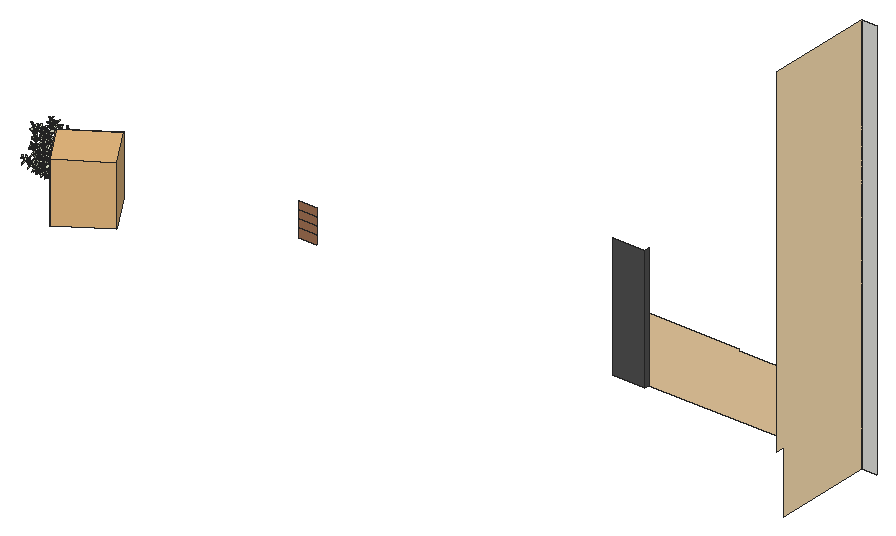
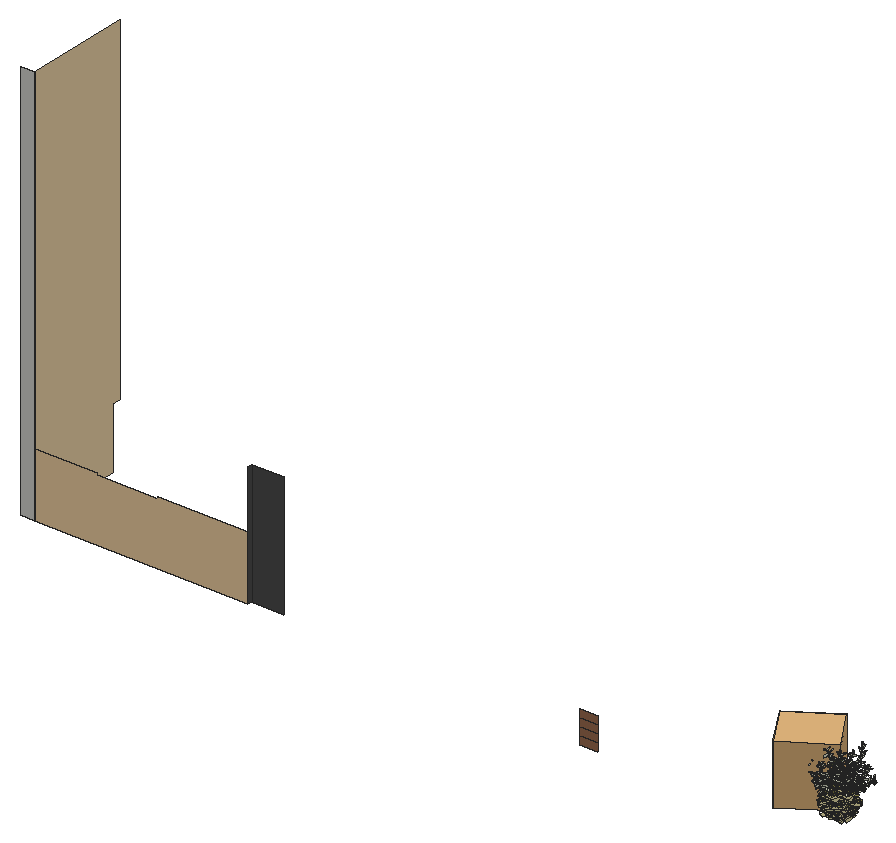
# SketchUp Ruby script. Lengths in inches.
U = 1.inch
M = Sketchup.active_model
def pt(a) = Geom::Point3d.new(a.map { |v| v * U })
def face(e, loops, mat)
  f = e.add_face(loops[0].map { |a| pt(a) })
  loops[1..].each { |l| e.add_face(l.map { |a| pt(a) }).erase! }
  f.material = f.back_material = mat if mat
  f
end
# faces: each face lists its corners as indices into pts; further lists are holes
def faces(e, pts, list, mat = nil) = list.each { |f| face(e, (f[0].is_a?(Array) ? f : [f]).map { |l| l.map { |i| pts[i] } }, mat) }
# xy, xz, yz: faces in a plane at the given z, y or x. An outline is a flat list of corners, or four numbers for a rectangle; further outlines are holes
def ring(l) = l.size == 4 ? [[l[0], l[1]], [l[2], l[1]], [l[2], l[3]], [l[0], l[3]]] : l.each_slice(2).to_a
def flat(e, list, mat, &to3) = list.each { |f| face(e, (f[0].is_a?(Array) ? f : [f]).map { |l| ring(l).map { |u, v| to3.(u, v) } }, mat) }
def xy(e, z, list, mat = nil) = flat(e, list, mat) { |x, y| [x, y, z] }
def xz(e, y, list, mat = nil) = flat(e, list, mat) { |x, z| [x, y, z] }
def yz(e, x, list, mat = nil) = flat(e, list, mat) { |y, z| [x, y, z] }
def lines(e, pts, list) = list.each { |a, b| e.add_line(pt(pts[a]), pt(pts[b])) }
# prism: a flat outline (further loops are holes) pulled along v
def prism(e, loops, v, mat = nil)
  f = face(e, loops, mat); d = Geom::Vector3d.new(v.map { |x| x * U })
  f.pushpull(f.normal.samedirection?(d) ? d.length : -d.length)
end
def box(e, o, s, mat = nil) = prism(e, [[o, [o[0] + s[0], o[1], o[2]], [o[0] + s[0], o[1] + s[1], o[2]], [o[0], o[1] + s[1], o[2]]]], [0, 0, s[2]], mat)
def at(x, y, z, deg = 0) = Geom::Transformation.translation(pt([x, y, z])) * Geom::Transformation.rotation(ORIGIN, Z_AXIS, deg.degrees)
def axes(o, x, y, z) = Geom::Transformation.new([*x, 0, *y, 0, *z, 0, *pt(o).to_a, 1])
def part(name) = M.definitions.add(name)
# library, detail: a bought-in or finely detailed component or shape, given as its bounding box
def library(name, o, s) = part(name).tap { |d| box(d.entities, o, s) }
def detail(e, o, s) = box(e.add_group.entities, o, s)
def put(e, d, t, mat = nil) = e.add_instance(d, t).tap { |i| i.material = mat if mat }
def group(e, t, mat = nil) = e.add_group.tap { |g| g.transformation = t; g.material = mat if mat }.entities
root = M.entities
M.materials.add("0ad16as01f6asdLeafVar1sfd015as60f1as6").color = [231, 235, 211]
M.materials.add("Colorsadfasdfa0sd1f06w3").color = [153, 130, 61]
M.materials.add("Euphorbia asdfasd0f150160s159w").color = [180, 173, 131]
M.materials.add("Euphorbiaasdfa0sdf1a56sd016wow Leaf SU").color = [141, 134, 72]
M.materials.add("[0032_Moccasin]").color = [255, 228, 181]
M.materials.add("[0033_NavajoWhite]").color = [255, 222, 173]
M.materials.add("[0135_DarkGray]").color = [81, 81, 81]
M.materials.add("[Tile Ceramic Multi]").color = [165, 115, 84]
M.materials.add("asdfasdf0165f6asdLeafVar1sfd015as60f1as6").color = [231, 235, 211]
M.materials.add("dw_stemssadfasdfa0sdf1s01d6w1").color = [90, 97, 50]
M.materials.add("viburnumbladsadfasdfad0w122").color = [125, 129, 119]
c1 = part("Component\#315")
p = [[0.25,0,0],[2.05,0.01,0.35],[1.81,4.2,1.66],[0,4.19,1.3125]]
faces(c1.entities,p,[[0,1,2,3]],"viburnumbladsadfasdfad0w122")
c2 = part("viburnumblad2")
put(c2.entities,c1,axes([-19.23,-4.49,-32.18],[83.35428,0,0],[0,79.38502,0],[0,0,83.35428]))
c3 = part("vdw_leaf\#2")
p = [[0,0,0],[-2.77,1.61,2.32],[-4.3125,6.1,4.5],[-3.97,13.49,6.09],[-2.47,18.57,6.3],[-0.2,22.73,5.75],
  [2.54,19.66,6.85],[4.3,15.93,7.09],[5.03,7.6,5.43],[3.32,1.76,2.74]]
faces(c3.entities,p,[[0,1,2,3,4,5],[0,5,6,7,8,9]],"asdfasdf0165f6asdLeafVar1sfd015as60f1as6")
c4 = part("dg_branch_1\#2")
p = [[46.12,1.57,35.62],[46,5.42,35.41],[0.14,1.79,0.05],[0.26,-2.0625,0.27],[74.05,2.99,75.8],[74.11,5.28,75.58],
  [103.46,0.47,94.74],[104.03,2.92,94.84],[81.14,16.92,120.46],[81.2,18.78,120.24],[130.47,-5.6875,130.27],[130.58,-3.66,129.85],
  [80.82,34.4375,191.22],[80.64,35.93,190.9],[148.49,-14.56,203.24],[148.9,-12.8125,203.11],[81.08,37.95,226.93],[81.4,39.1,227.03],
  [157.45,-18.19,250.77],[157.7,-17.01,250.41]]
faces(c4.entities,p,[[0,1,2,3],[4,0,1],[4,1,5],[6,4,5],[6,5,7],[8,4,5],[8,5,9],[10,6,7],
  [10,7,11],[12,8,9],[12,9,13],[14,10,11],[14,11,15],[16,12,13],[16,13,17],[18,14,15],
  [18,15,19]],"dw_stemssadfasdfa0sdf1s01d6w1")
c5 = part("vdw_branch1\#3")
put(c5.entities,c3,axes([120.69,-2.42,117.31],[1.12221,-0.24063,-0.65809],[0.19207,1.24776,-0.12871],[0.65778,0.01392,1.11658]))
put(c5.entities,c3,axes([81,38.9,226.05],[0.7888,-0.58155,0],[0.48308,0.65523,0.47],[-0.28484,-0.38635,0.83138]))
put(c5.entities,c3,axes([78.08,12.69,106.05],[-1.43826,-0.02353,-0.03177],[0.0088,-1.31777,0.57755],[-0.03854,0.57714,1.31741]))
put(c5.entities,c3,axes([130.18,-4.73,130.41],[-0.38031,-1.29044,-0.11242],[1.20662,-0.31032,-0.51987],[0.47109,-0.24694,1.24081]))
put(c5.entities,c3,axes([157.08,-17.89,249.93],[-0.91355,0.40674,0],[-0.37496,-0.84216,0.38752],[0.15762,0.35401,0.92186]))
put(c5.entities,c3,axes([90.64,3.03,86.49],[0.32514,-0.85045,-0.99675],[0.69523,0.98247,-0.61148],[1.11061,-0.36604,0.67459]))
put(c5.entities,c3,axes([80.15,28.42,160.95],[-0.16039,0.95636,-1.06292],[-1.41646,0.03966,0.24943],[0.19509,1.07422,0.93709]))
put(c5.entities,c3,axes([126.74,-5.45,129.22],[-0.59819,0.96152,-0.6841],[-0.85772,0.12575,0.92675],[0.75427,0.88089,0.57856]))
put(c5.entities,c3,axes([133.22,-6.12,150.66],[-0.93823,0.76985,0.59124],[-0.47726,-1.08188,0.65135],[0.84525,0.24366,1.02405]))
put(c5.entities,c3,axes([80.43,22.89,141.32],[-1.42571,-0.19312,0.01373],[0.18338,-1.31425,0.5561],[-0.0621,0.5528,1.32692]))
put(c5.entities,c3,axes([33.14,0.88,26.42],[-0.13338,1.31536,0.04876],[-1.04528,-0.13221,0.7073],[0.72315,0.03348,1.07497]))
put(c5.entities,c3,axes([152.63,-15.08,221.76],[-1.28188,0.41945,0.0579],[-0.3638,-1.18547,0.53367],[0.21665,0.49113,1.23869]))
put(c5.entities,c3,axes([80.05,28.28,160.33],[-0.46732,-1.26661,0.40679],[1.27397,-0.40257,0.21004],[-0.07408,0.44645,1.30501]))
put(c5.entities,c3,axes([153.95,-14.8,235.875],[0.39005,1.07743,0.20605],[-0.96443,0.25296,0.50293],[0.42961,-0.3464,0.99807]))
put(c5.entities,c3,axes([80.2,24.22,141.74],[1.33062,-0.46576,0.02628],[0.44746,1.2746,-0.06608],[-0.00197,0.0722,1.37936]))
put(c5.entities,c3,axes([145.48,-12.5,188.92],[-1.32952,0.16983,0.16138],[-0.09299,-1.2361,0.53471],[0.21503,0.51548,1.22904]))
put(c5.entities,c3,axes([139.64,-9.18,171.24],[0.05682,1.30088,0.23414],[-1.13176,-0.05343,0.57151],[0.58357,-0.22963,1.13417]))
put(c5.entities,c3,axes([70.95,4.35,71.98],[-1.1081,-0.41873,0.64752],[0.33675,-1.28259,-0.25313],[0.6937,-0.04625,1.15721]))
put(c5.entities,c3,axes([59.85,4.55,56.17],[-0.26797,1.24526,0.35754],[-0.9369,-0.41634,0.74783],[0.83377,-0.10389,0.98674]))
put(c5.entities,c3,axes([33.11,3.36,25.66],[-0.57817,-1.07968,-0.5679],[1.11554,-0.21356,-0.7297],[0.49375,-0.78178,0.98363]))
put(c5.entities,c4,at(-0.21,0.34,-0.17),"dw_stemssadfasdfa0sdf1s01d6w1")
put(c5.entities,c3,axes([80.91,19.01,122.53],[-0.84258,1.13222,-0.27981],[-1.15093,-0.75138,0.42537],[0.18861,0.47293,1.3457]))
put(c5.entities,c3,axes([119.8,-1.22,114.1],[-1.3235,-0.25012,0.09101],[0.25933,-1.31572,0.15537],[0.05991,0.1698,1.33794]))
put(c5.entities,c3,axes([46.29,5.1,38.04],[0.98937,0.73827,-0.47585],[-0.72359,1.03721,0.10473],[0.44068,0.18581,1.20453]))
put(c5.entities,c3,axes([81.1875,33.03,184.45],[1.33883,0.26986,0.35053],[-0.09581,1.22087,-0.57399],[-0.42216,0.53228,1.20262]))
put(c5.entities,c3,axes([80.16,36.28,206.98],[-0.83993,0.85737,-0.6234],[-1.05964,-0.65701,0.5241],[0.02941,0.81391,1.07976]))
put(c5.entities,c3,axes([154.86,-16.15,234.87],[0.02509,-1.15302,-0.28506],[1.1487,-0.04894,0.29908],[-0.30202,-0.28195,1.11384]))
put(c5.entities,c3,axes([108.77,-0.33,101.14],[-0.47691,-1.03266,-0.72709],[1.25395,-0.29455,-0.40416],[0.15052,-0.81814,1.06325]))
put(c5.entities,c3,axes([89.79,3.01,85.87],[-0.61344,0.75518,0.8965],[-0.17758,-1.01824,0.73622],[1.13385,0.22574,0.58569]))
put(c5.entities,c3,axes([81.56,20.31,123.29],[0.37259,-1.3435,0.21057],[1.29385,0.32364,-0.22445],[0.16906,0.25791,1.34638]))
put(c5.entities,c3,axes([46.45,1.82,36.74],[-0.77883,0.29892,1.0614],[0.19124,-1.24314,0.49044],[1.08598,0.43329,0.67484]))
put(c5.entities,c3,axes([71.37,4.02,72.32],[0.72905,0.81546,-0.74421],[-0.66805,0.98958,0.42988],[0.8391,0.14186,0.97745]))
put(c5.entities,c3,axes([136.59,-5.88,150.53],[0.85845,-0.99897,-0.12437],[0.96526,0.81273,0.13453],[-0.02572,-0.18182,1.28292]))
put(c5.entities,c3,axes([80.375,38.8,225.86],[-0.25178,0.96778,0],[-0.89216,-0.23211,0.38752],[0.37503,0.09757,0.92186]))
put(c5.entities,c3,axes([74.43,7.99,85.38],[-1.05703,0.91669,-0.33543],[-0.95806,-0.87958,0.61531],[0.18697,0.6754,1.25659]))
put(c5.entities,c3,axes([76.57,9.74,89.32],[0.63146,-1.21538,0.33508],[1.18148,0.49387,-0.43517],[0.26321,0.48577,1.26593]))
put(c5.entities,c3,axes([81.6875,36.97,207.4],[0.09422,-1.04424,0.38486],[1.01646,0.1939,0.27727],[-0.33299,0.33382,0.98727]))
put(c5.entities,c3,axes([157.29,-17.17,249.98],[0.50586,-0.50586,0],[0.38853,0.38853,0.41105],[-0.29684,-0.29684,0.56115]))
put(c5.entities,c3,axes([79.92,15.8,106.09],[1.03917,-0.29343,-0.90675],[-0.14587,1.22131,-0.5624],[0.92163,0.5191,0.88824]))
put(c5.entities,c3,axes([61.95,3.88,56.26],[0.41243,-1.28546,0],[1.17466,0.37688,-0.54831],[0.5221,0.16751,1.23363]))
put(c5.entities,c3,axes([151.99,-14.79,208.15],[-0.48571,-1.21723,-0.32393],[1.25386,-0.50033,0],[-0.12005,-0.30087,1.31056]))
put(c5.entities,c3,axes([108.44,0.62,102.22],[0.82183,0.96078,0.38967],[-0.62327,0.08618,1.10203],[0.79141,-0.88661,0.51693]))
put(c5.entities,c3,axes([145.6,-10.56,188.62],[1.03241,-0.02554,-0.82693],[0.3944,1.11584,0.45794],[0.70325,-0.61672,0.89706]))
put(c5.entities,c3,axes([78.59,32.3,183.89],[-1.12675,-0.42036,0.43987],[0.5899,-0.98149,0.57312],[0.14901,0.70693,1.05726]))
put(c5.entities,c3,axes([152.08,-13.42,223.37],[0.79993,-0.44251,-0.69938],[0.68456,0.82615,0.26026],[0.41048,-0.60953,0.85515]))
put(c5.entities,c3,axes([140.71,-8.74,170.55],[0.41903,-1.24177,-0.32393],[1.26224,0.33728,0.33986],[-0.23168,-0.40836,1.26573]))
put(c5.entities,c3,axes([149.25,-12.53,205.78],[1.24456,0.38285,0.23414],[-0.42999,1.04826,0.57151],[-0.02056,-0.62679,1.13417]))
c6 = part("vdw_leaf\#3")
p = [[0,0,0],[-2.77,1.61,2.32],[-4.3125,6.1,4.5],[-3.97,13.49,6.09],[-2.47,18.57,6.3],[-0.2,22.73,5.75],
  [2.54,19.66,6.85],[4.3,15.93,7.09],[5.03,7.6,5.43],[3.32,1.76,2.74]]
faces(c6.entities,p,[[0,1,2,3,4,5],[0,5,6,7,8,9]],"asdfasdf0165f6asdLeafVar1sfd015as60f1as6")
c7 = part("dw_brancj_2\#2")
p = [[9.7,-0.22,29.95],[0.23,-1.96,0.34],[-0.05,1.51,0.11],[9.65,1.51,29.46],[18.64,-8.75,84.43],[18.96,-6.63,84.625],
  [1.53,6.02,63.68],[1.42,8.18,63.25],[-10.58,8.77,161.17],[-10.41,9.98,160.68],[26.34,-9.37,211.72],[26.57,-8.28,211.23]]
faces(c7.entities,p,[[0,1,2],[0,2,3],[4,0,3],[4,3,5],[6,0,3],[6,3,7],[8,6,7],[8,7,9],
  [10,4,5],[10,5,11]],"dw_stemssadfasdfa0sdf1s01d6w1")
c8 = part("vdw_branch2\#3")
put(c8.entities,c6,axes([19.53,-5.9,102.42],[1.12377,-0.50004,0],[0.46097,1.03596,0.47664],[-0.19377,-0.43548,1.13389]))
put(c8.entities,c6,axes([-5.89,6.52,109.44],[-1.07209,0.83679,0],[-0.77141,-0.98832,0.52702],[0.32427,0.41545,1.25373]))
put(c8.entities,c6,axes([-0.44,8.23,75.28],[0.88709,-0.9947,0],[0.92159,0.82189,0.33087],[-0.25219,-0.22491,1.26111]))
put(c8.entities,c6,axes([24.71,-8.97,190.81],[-0.82641,0.91101,0],[-0.83983,-0.76184,0.47664],[0.35303,0.32025,1.13389]))
put(c8.entities,c6,axes([-2.29,8.24,91.35],[1.24603,-0.47303,0],[0.43826,1.15445,0.33087],[-0.11993,-0.31592,1.26111]))
put(c8.entities,c6,axes([12.26,-3.11,37.92],[-0.64625,1.02205,0.22511],[-1.04383,-0.61044,-0.22511],[-0.07533,-0.30931,1.18809]))
put(c8.entities,c6,axes([26.17,-9.17,210.27],[-0.99452,-0.10453,0],[0.09636,-0.91681,0.38752],[-0.04051,0.38539,0.92186]))
put(c8.entities,c6,axes([-6.07,9.4,125.35],[-0.90214,-0.98107,0],[0.90896,-0.83583,0.33087],[-0.24874,0.22873,1.26111]))
put(c8.entities,c6,axes([-4.13,7.29,110.58],[0.44715,-1.078,0.64369],[1.05816,0.63649,0.33087],[-0.58725,0.40856,1.09216]))
put(c8.entities,c6,axes([23.91,-8.22,171.96],[0.62307,0.85009,-0.63406],[-0.71531,0.8798,0.47664],[0.78296,0.12729,0.94004]))
put(c8.entities,c7,at(-0.09,0.18,-0.25),"dw_stemssadfasdfa0sdf1s01d6w1")
put(c8.entities,c6,axes([23.34,-9.65,156.59],[-0.31364,-1.00782,0.58216],[1.10369,-0.17062,0.29925],[-0.17137,0.6239,0.98776]))
put(c8.entities,c6,axes([15.03,-3.37,58.83],[-1.05425,-0.00194,0.58442],[-0.14303,-1.11707,-0.26172],[0.55355,-0.3046,0.99755]))
put(c8.entities,c6,axes([-11.625,9.46,160.37],[0.36812,0.92978,0],[-0.85713,0.33936,0.38752],[0.3603,-0.14265,0.92186]))
put(c8.entities,c6,axes([21.32,-8.53,138.72],[1.21379,0.19904,0],[-0.19904,1.21379,0],[0,0,1.23]))
put(c8.entities,c6,axes([22.54,-9.2,141.43],[-1.02887,0.17955,0.60182],[-0.23387,-1.13057,-0.06253],[0.56696,-0.17376,1.02111]))
put(c8.entities,c6,axes([23.9,-8.82,173.84],[-1.14567,-0.37474,0],[0.35918,-1.0981,0.04438],[-0.01409,0.04308,1.17993]))
put(c8.entities,c6,axes([-7.84,8.92,143.59],[-1.26971,0.40522,0],[-0.37543,-1.17638,0.33087],[0.10274,0.32192,1.26111]))
put(c8.entities,c6,axes([19.77,-8.01,85.98],[-0.32405,-1.14591,0.18674],[1.10278,-0.32969,-0.10948],[0.15845,0.14442,1.16117]))
put(c8.entities,c6,axes([-0.62,5.76,76.34],[-0.08879,1.17576,-0.67771],[-1.34525,-0.16582,-0.11144],[-0.17897,0.66309,1.17383]))
put(c8.entities,c6,axes([20.49,-8.22,121.07],[0.39924,-0.78471,-0.8233],[1.08735,0.33121,0.2116],[0.09035,-0.83005,0.83495]))
put(c8.entities,c6,axes([15.15,-3.72,62.9],[1.16251,0.40128,-0.0211],[-0.39924,1.16074,0.07874],[0.0456,-0.06757,1.2273]))
put(c8.entities,c6,axes([20.72,-8.08,120.26],[-0.03693,1.2277,-0.06551],[-1.22944,-0.03698,0],[-0.00197,0.06548,1.22825]))
put(c8.entities,c6,axes([22.58,-8.36,155.57],[-0.56247,1.09386,0],[-1.00839,-0.51852,0.47664],[0.42389,0.21796,1.13389]))
put(c8.entities,c6,axes([3.97,3.13,57.96],[-1.09459,0.76041,0],[-0.72262,-1.0402,-0.1735],[-0.10109,-0.14552,1.29352]))
put(c8.entities,c6,axes([-10.8,9.06,160.75],[-0.66334,-0.72138,0],[0.66835,-0.61458,0.24329],[-0.1829,0.16818,0.92729]))
put(c8.entities,c6,axes([19.06,-9.3125,103.96],[-1.01345,0.25553,-0.60051],[-0.2265,-1.12952,-0.09839],[-0.59598,0.03076,1.01889]))
put(c8.entities,c6,axes([18.07,-6.2,81.7],[-0.56247,1.09386,0],[-1.00839,-0.51852,0.47664],[0.42389,0.21796,1.13389]))
put(c8.entities,c6,axes([12.95,-0.39,43.31],[0.13044,-1.19832,0],[1.11025,0.12085,0.29925],[-0.30382,-0.03307,1.14057]))
put(c8.entities,c6,axes([2.28,8.28,56.18],[1.32413,-0.31027,0],[0.30923,1.31968,-0.11144],[0.02542,0.1085,1.35543]))
put(c8.entities,c6,axes([-7.55,9.96,143.07],[1.34251,-0.21744,0],[0.20045,1.23761,0.52702],[-0.08426,-0.52024,1.25373]))
put(c8.entities,c6,axes([26.15,-8.25,210.66],[0.94661,-0.25364,0],[0.235,0.87703,0.24329],[-0.06431,-0.24,0.92729]))
put(c8.entities,c6,axes([-6.48,11.37,125.16],[0.64635,1.10315,0.46356],[-1.16569,0.46153,0.52702],[0.27017,-0.6478,1.16488]))
put(c8.entities,c6,axes([25.74,-8.35,191.28],[0.13044,-1.19832,0],[1.11025,0.12085,0.29925],[-0.30382,-0.03307,1.14057]))
put(c8.entities,c6,axes([-5.125,7.47,91.6],[-1.10024,0.63688,0.48318],[-0.78682,-1.00808,-0.46292],[0.14137,-0.65404,1.184]))
c9 = part("Component\#306")
p = [[4.55,0.11,0],[4.55,0,0],[2.84,0,3.13],[2.84,0.11,3.13],[4.625,0.05,0.04],[2.92,0.05,3.15],
  [2.08,0,8.07],[2.08,0.11,8.07],[2.16,0.05,8.1],[0,0,12.54],[0,0.11,12.54],[0.07,0.05,12.58]]
faces(c9.entities,p,[[0,1,2,3],[1,4,5,2],[1,0,4],[4,0,3,5],[3,2,6,7],[2,5,8,6],[5,3,7,8],[7,6,9,10],
  [6,8,11,9],[8,7,10,11],[10,9,11]],"Colorsadfasdfa0sd1f06w3")
c10 = part("Component\#301")
xy(c10.entities,0,[[0,0,0.7,3.1]],"Euphorbiaasdfa0sdf1a56sd016wow Leaf SU")
c11 = part("Leaf rosette")
put(c11.entities,c10,axes([2.21,1.74,0.13],[-0.4441,0.47879,-0.0956],[-0.4878,-0.4406,0.05935],[-0.03146,0.16757,0.98536]))
put(c11.entities,c10,axes([2.29,1.9,0.17],[-0.62678,-0.10063,-0.18061],[0.01105,-0.59203,0.2915],[-0.31282,0.41486,0.85442]))
put(c11.entities,c10,axes([2.09,1.69,0.1],[-0.10438,0.65169,0],[-0.65169,-0.10438,0],[0,0,1]))
put(c11.entities,c10,axes([1.97,1.77,0.02],[0.31114,0.5228,0.25587],[-0.57125,0.32993,0.02052],[-0.16918,-0.3502,0.92127]))
put(c11.entities,c10,axes([1.93,1.95,0],[0.54816,-0.03215,0.36617],[-0.11878,0.60671,0.23108],[-0.52706,-0.39065,0.75472]))
put(c11.entities,c10,axes([2.04,2.1,0.05],[0.26275,-0.55867,0.23335],[0.34186,0.34684,0.44545],[-0.75711,-0.08556,0.64766]))
put(c11.entities,c10,axes([2.22,2.08,0.13],[-0.29265,-0.59104,-0.02512],[0.40323,-0.2198,0.47401],[-0.65583,0.2952,0.69479]))
c12 = part("Component\#308")
xy(c12.entities,0,[[0,0,5.01,4.64]],"Euphorbia asdfasd0f150160s159w")
c13 = part("Component\#316")
put(c13.entities,c9,at(2.35,3.5,0))
put(c13.entities,c11,at(0.25,1.59,12.45))
put(c13.entities,c12,axes([7.46,0.77,3.64],[0.10848,0.99337,0.03799],[-0.82378,0.11122,-0.55589],[-0.55643,0.02901,0.83038]))
put(c13.entities,c12,axes([1.97,2.58,1.93],[0.80762,-0.50565,0.30344],[0.47433,0.86274,0.17519],[-0.35038,0.00244,0.93661]))
put(c13.entities,c12,axes([5.79,0.14,3.9],[0.5013,0.78918,0.35482],[-0.74775,0.60146,-0.2813],[-0.4354,-0.1243,0.89162]))
put(c13.entities,c12,axes([1.87,2.6,3.75],[0.73154,-0.49698,0.46676],[0.47433,0.86274,0.17519],[-0.48976,0.09324,0.86686]))
put(c13.entities,c12,axes([3.91,7.06,6.66],[-0.50827,-0.83837,-0.19699],[0.8278,-0.53869,0.15675],[-0.23753,-0.08339,0.96779]))
put(c13.entities,c12,axes([1.2,3.99,6.83],[0.56066,-0.79708,0.22433],[0.74237,0.60386,0.29025],[-0.36682,0.0038,0.93028]))
put(c13.entities,c10,axes([2.42,3.73,12.57],[-0.1322,-0.64472,0.04955],[0.10064,0.02944,0.65162],[-0.9678,0.2092,0.14002]))
put(c13.entities,c10,axes([2.57,3.43,12.63],[-0.62833,0.089,-0.18134],[-0.19954,-0.36568,0.51192],[-0.04764,0.82148,0.56824]))
put(c13.entities,c12,axes([4.04,6.92,11.09],[-0.67411,-0.5063,-0.5378],[0.44628,-0.85937,0.24964],[-0.58857,-0.07172,0.80526]))
put(c13.entities,c10,axes([2.5,3.49,12.74],[-0.62833,0.089,-0.18134],[-0.18746,-0.03618,0.63178],[0.11402,0.98935,0.09049]))
put(c13.entities,c10,axes([2.3,3.27,12.51],[0.02916,0.64747,0.12464],[-0.56235,-0.04072,0.34308],[0.5216,-0.18387,0.83314]))
put(c13.entities,c12,axes([0.26,4.96,9.69],[0.33661,-0.92735,0.16343],[0.73504,0.36725,0.56995],[-0.58857,-0.07172,0.80526]))
put(c13.entities,c12,axes([4.76,6.31,12.62],[-0.95056,-0.1129,-0.28929],[0.09021,-0.99179,0.09066],[-0.29715,0.06008,0.95294]))
put(c13.entities,c12,axes([5.2,6.55,10.37],[-0.76372,-0.27738,-0.58291],[0.26517,-0.95808,0.10848],[-0.58857,-0.07172,0.80526]))
c14 = part("Plant stem")
p = [[2.84,0.11,3.13],[2.84,0,3.13],[2.08,0,8.07],[2.08,0.11,8.07],[2.92,0.05,3.15],[2.16,0.05,8.1],
  [0,0,12.54],[0,0.11,12.54],[0.07,0.05,12.58]]
faces(c14.entities,p,[[0,1,2,3],[1,4,5,2],[4,0,3,5],[3,2,6,7],[2,5,8,6],[5,3,7,8],[7,6,8]],"Colorsadfasdfa0sd1f06w3")
c15 = part("Leafy shoot")
put(c15.entities,c14,at(2.35,3.5,0))
put(c15.entities,c11,at(0.25,1.59,12.45))
put(c15.entities,c12,axes([1.87,2.6,3.75],[0.73154,-0.49698,0.46676],[0.47433,0.86274,0.17519],[-0.48976,0.09324,0.86686]))
put(c15.entities,c12,axes([3.91,7.06,6.66],[-0.50827,-0.83837,-0.19699],[0.8278,-0.53869,0.15675],[-0.23753,-0.08339,0.96779]))
put(c15.entities,c12,axes([1.2,3.99,6.83],[0.56066,-0.79708,0.22433],[0.74237,0.60386,0.29025],[-0.36682,0.0038,0.93028]))
put(c15.entities,c10,axes([2.42,3.73,12.57],[-0.1322,-0.64472,0.04955],[0.10064,0.02944,0.65162],[-0.9678,0.2092,0.14002]))
put(c15.entities,c10,axes([2.57,3.43,12.63],[-0.62833,0.089,-0.18134],[-0.19954,-0.36568,0.51192],[-0.04764,0.82148,0.56824]))
put(c15.entities,c12,axes([4.04,6.92,11.09],[-0.67411,-0.5063,-0.5378],[0.44628,-0.85937,0.24964],[-0.58857,-0.07172,0.80526]))
put(c15.entities,c10,axes([2.5,3.49,12.74],[-0.62833,0.089,-0.18134],[-0.18746,-0.03618,0.63178],[0.11402,0.98935,0.09049]))
put(c15.entities,c10,axes([2.3,3.27,12.51],[0.02916,0.64747,0.12464],[-0.56235,-0.04072,0.34308],[0.5216,-0.18387,0.83314]))
put(c15.entities,c12,axes([0.26,4.96,9.69],[0.33661,-0.92735,0.16343],[0.73504,0.36725,0.56995],[-0.58857,-0.07172,0.80526]))
put(c15.entities,c12,axes([4.76,6.31,12.62],[-0.95056,-0.1129,-0.28929],[0.09021,-0.99179,0.09066],[-0.29715,0.06008,0.95294]))
put(c15.entities,c12,axes([5.2,6.55,10.37],[-0.76372,-0.27738,-0.58291],[0.26517,-0.95808,0.10848],[-0.58857,-0.07172,0.80526]))
put(c15.entities,c12,axes([7.03,0.77,3.77],[0.19714,0.84663,0.32426],[-0.94994,0.28899,-0.30484],[-0.2731,-0.45173,0.91532]))
c16 = part("Groundcover plant")
put(c16.entities,c13,axes([0.82,1.83,0.8125],[0.98541,0,-0.17021],[0,1,0],[0.17021,0,0.98541]))
put(c16.entities,c15,axes([4.45,-0.84,-2.24],[0.69527,0.50616,0],[-0.50264,0.69042,-0.10135],[-0.05965,0.08194,0.85401]))
put(c16.entities,c15,axes([1.85,7.37,-3.38],[0.7038,-0.47341,0.14191],[0.46407,0.71797,0.09357],[-0.16999,0,0.84303]))
put(c16.entities,c15,axes([6.9,-3.65,-2.52],[0.79351,0.57769,0],[-0.57366,0.78798,-0.11567],[-0.06808,0.09351,0.97468]))
put(c16.entities,c15,axes([1.36,5.18,-2.66],[0.50674,-0.34086,0.10218],[0.33413,0.51694,0.06737],[-0.12239,0,0.60698]))
put(c16.entities,c15,axes([5.76,-1.49,-2.17],[0.43479,0.43181,0.07251],[-0.43488,0.43544,-0.06951],[-0.06212,-0.06169,0.61918]))
c17 = part("Groundcover clump")
put(c17.entities,c16,axes([25.06,6.72,0.82],[-0.74291,1.22188,0],[-1.22188,-0.74291,0],[0,0,1]))
put(c17.entities,c16,axes([-0.76,2.1875,0.82],[1.43,0,0],[0,1.43,0],[0,0,1]))
put(c17.entities,c16,axes([8.21,24.79,0.82],[-0.6403,-1.27864,0],[1.27864,-0.6403,0],[0,0,1]))
c18 = part("vdw_leaf\#1")
p = [[0,0,0],[-2.77,1.61,2.32],[-4.3125,6.1,4.5],[-3.97,13.49,6.09],[-2.47,18.57,6.3],[-0.2,22.73,5.75],
  [2.54,19.66,6.85],[4.3,15.93,7.09],[5.03,7.6,5.43],[3.32,1.76,2.74]]
faces(c18.entities,p,[[0,1,2,3,4,5],[0,5,6,7,8,9]],"0ad16as01f6asdLeafVar1sfd015as60f1as6")
c19 = part("dw_branch_3\#2")
p = [[-10.06,-1.6,62.9],[-0.2,1.54,-0.01],[-10.43,1.54,62.72],[0.18,-1.6,0.17],[-23.75,-21.66,88.91],[-25.7,-20.3,89.55],
  [13.4,11.62,104.56],[13.33,13.52,104.47],[-49.25,-41.87,130.3125],[-50.33,-40.21,130.71],[-4.97,21.13,143.98],[35.61,27.99,178.64],
  [-5.09,23.64,143.96],[35.32,29.14,178.46],[-67.7,-55.38,181.06],[-68.34,-54.45,181.62],[-22.8125,33.9,200.59],[-22.94,35.79,200.41],
  [56.61,36.78,229.75],[56.29,38.09,229.57],[-70.63,-67.46,248.85],[-70.72,-66.33,249.5],[-25.05,43.32,240.75],[-24.98,44.26,240.57]]
faces(c19.entities,p,[[0,1,2],[0,3,1],[4,2,5],[4,0,2],[6,0,2],[6,2,7],[8,4,5],[8,5,9],
  [10,6,7],[11,6,7],[10,7,12],[11,7,13],[14,8,9],[14,9,15],[16,10,12],[16,12,17],
  [18,11,13],[18,13,19],[20,14,15],[20,15,21],[22,16,17],[22,17,23]],"dw_stemssadfasdfa0sdf1s01d6w1")
c20 = part("dw_branch3\#2")
put(c20.entities,c18,axes([-70.33,-63.58,233.32],[-1.00752,0.412,0.78596],[-0.24851,-1.22189,0.32195],[0.83141,0.09817,1.01433]))
put(c20.entities,c18,axes([-66.93,-54.91,182.82],[-0.84976,-0.98359,0.33619],[0.99572,-0.74889,0.32577],[-0.05223,0.46521,1.22907]))
put(c20.entities,c18,axes([-46.12,-39.49,126.35],[1.23843,0.5364,0.23552],[-0.56438,0.94474,0.81599],[0.15707,-0.83465,1.07498]))
put(c20.entities,c18,axes([13.0625,13.13,104.77],[-1.01271,0.69982,-0.26884],[-0.74268,-0.99813,0.19939],[-0.10222,0.31872,1.21473]))
put(c20.entities,c18,axes([-18.87,30.42,186.42],[0.36309,1.06515,-0.56675],[-1.14134,0.49515,0.19939],[0.39128,0.45593,1.10754]))
put(c20.entities,c18,axes([-3.2,4.15,75.77],[-1.04153,0.55414,0.44243],[-0.23365,-1.01045,0.71554],[0.6695,0.50943,0.93801]))
put(c20.entities,c18,axes([23.2,19.41,136.3],[-0.65687,-1.11295,-0.05714],[1.05857,-0.61429,-0.20411],[0.15163,-0.1536,1.24868]))
put(c20.entities,c18,axes([-25.57,35.48,201.32],[-0.64726,0.62827,0.87973],[-0.71635,-1.0172,0.19939],[0.80962,-0.39773,0.87973]))
put(c20.entities,c18,axes([-36.37,-32.14,110.35],[-0.80747,1.09962,0.12544],[-0.83333,-0.50188,-0.96467],[-0.72833,-0.64487,0.96467]))
put(c20.entities,c18,axes([-9.89,26.72,156.79],[0.45529,1.02969,0.56572],[-1.16919,0.33753,0.32662],[0.11537,-0.64297,1.07744]))
put(c20.entities,c18,axes([-26.57,46.1,241.0625],[0.00015,0.80921,0.22536],[-0.83985,0.00446,-0.01542],[-0.01605,-0.22532,0.80906]))
put(c20.entities,c18,axes([-9.2,-2.58,61.06],[-1.10001,-0.40312,0.39014],[0.40883,-1.1116,0.00411],[0.35732,0.13566,1.14763]))
put(c20.entities,c18,axes([-69.91,-63.11,233.93],[1.36249,-0.1432,0],[0.13201,1.25603,0.5309],[-0.05549,-0.52799,1.26295]))
put(c20.entities,c18,axes([32.2,25.46,166.13],[0.06878,-1.29051,-0.05714],[1.22165,0.07415,-0.20411],[0.2113,-0.04403,1.24868]))
put(c20.entities,c18,axes([-5.68,-0.66,44.43],[-0.48448,-1.12287,0.17078],[0.98138,-0.33653,0.57135],[-0.48308,0.36756,1.04626]))
put(c20.entities,c18,axes([43.45,32.81,198.64],[0.5408,1.19584,0.14106],[-0.94242,0.32409,0.86557],[0.74952,-0.45533,0.98656]))
put(c20.entities,c18,axes([12.52,14.14,104.98],[1.02694,0.54888,0.41092],[-0.53566,1.05407,-0.06927],[-0.38969,-0.12321,1.13846]))
put(c20.entities,c18,axes([44.55,32.375,198.73],[-0.65687,-1.11295,-0.05714],[1.05857,-0.61429,-0.20411],[0.15163,-0.1536,1.24868]))
put(c20.entities,c18,axes([-5.67,21.17,141.44],[-1.10726,0.43603,-0.32953],[-0.49537,-1.03435,0.29588],[-0.17521,0.40597,1.12589]))
put(c20.entities,c18,axes([55.69,37.84,229.48],[0.18984,0.96334,0.18958],[-0.71996,0.0053,0.69399],[0.66755,-0.26823,0.69457]))
put(c20.entities,c18,axes([-21.52,36.85,205.2],[0.72606,-0.98817,0.14519],[0.94364,0.7084,0.10251],[-0.16885,0.05176,1.19664]))
put(c20.entities,c18,axes([-68.51,-56.35,196.07],[1.16319,0.72381,0],[-0.66725,1.0723,0.5309],[0.28049,-0.45075,1.26295]))
put(c20.entities,c19,at(0.01,-0.09,-0.02),"dw_stemssadfasdfa0sdf1s01d6w1")
put(c20.entities,c18,axes([-2.49,5.18,75.91],[0.78614,-0.90346,-0.30078],[0.86953,0.79562,-0.11715],[0.28546,-0.14014,1.16705]))
put(c20.entities,c18,axes([-23.125,-16.22,82.25],[0.32175,1.32576,0.12544],[-1.33153,0.31835,0.05068],[0.01989,-0.13382,1.3633]))
put(c20.entities,c18,axes([-23.75,41.99,230.3],[0.85958,-0.87451,0.14519],[0.66531,0.75721,0.62192],[-0.54076,-0.36226,1.01955]))
put(c20.entities,c18,axes([27.07,22.48,149.34],[0.92952,-0.64745,-0.62467],[0.50188,1.074,-0.36637],[0.71693,0.02135,1.04468]))
put(c20.entities,c18,axes([17.66,16.25,119.93],[-0.91649,0.83891,-0.3601],[-0.87434,-0.77966,0.40896],[0.0492,0.54447,1.14321]))
put(c20.entities,c18,axes([-68.37,-54.54,181.63],[0.32047,1.28399,0.35434],[-1.33153,0.31835,0.05068],[-0.03484,-0.35624,1.32241]))
put(c20.entities,c18,axes([-28.98,-27.1,96.48],[-0.8814,-0.35966,-0.98523],[0.75246,-1.11336,-0.26672],[-0.73065,-0.71272,0.91382]))
put(c20.entities,c18,axes([-15.23,28.43,172.72],[-1.21149,0.11898,0.32517],[-0.09739,-1.25259,0.09551],[0.33228,0.0667,1.21356]))
put(c20.entities,c18,axes([-17.5625,31.23,186.85],[-0.49275,-1.12287,0.14519],[0.95014,-0.33653,0.62192],[-0.53717,0.36756,1.01955]))
put(c20.entities,c18,axes([26.7,21.22,149.39],[-1.00104,0.22334,0.83093],[0.36894,-1.0402,0.72406],[0.77731,0.78134,0.72643]))
put(c20.entities,c18,axes([-31.125,-24.87,97.38],[0.75482,-0.86936,0.69068],[-0.00159,0.80023,1.00899],[-1.08766,-0.58016,0.45842]))
put(c20.entities,c18,axes([-71.21,-66.73,248.67],[0.25207,0.96771,0],[-0.8921,0.23237,0.38752],[0.375,-0.09768,0.92186]))
put(c20.entities,c18,axes([-24.11,41.05,229.55],[-1.11612,0.51924,-0.26884],[-0.56394,-1.10897,0.19939],[-0.15444,0.29694,1.21473]))
put(c20.entities,c18,axes([6.75,8.37,91.63],[-0.33418,-1.12287,0.39014],[1.13558,-0.33653,0.00411],[0.10478,0.36756,1.14763]))
put(c20.entities,c18,axes([-26,45.89,241.63],[-0.26986,-0.70824,-0.32129],[0.56818,-0.39091,0.38449],[-0.49365,-0.09775,0.63011]))
put(c20.entities,c18,axes([3.74,17.32,124.35],[0.22441,1.22913,-0.16274],[-1.07812,0.11178,-0.64246],[-0.61228,0.25367,1.07162]))
put(c20.entities,c18,axes([-5.44,22.27,140.88],[1.2203,0.00475,0.31374],[-0.097,1.20386,0.35905],[-0.29841,-0.37189,1.1663]))
put(c20.entities,c18,axes([-13.79,29.35,173.31],[0.83169,-0.90108,0.14519],[0.68877,0.73594,0.62192],[-0.55187,-0.34509,1.01955]))
put(c20.entities,c18,axes([-16.92,-7.26,72.98],[1.30647,0.30378,-0.27886],[0.07026,0.74892,1.14503],[0.40633,-1.10623,0.69861]))
put(c20.entities,c18,axes([4.8,17.55,125.22],[-0.25598,-1.17842,0.26559],[1.01553,-0.08455,0.60363],[-0.56975,0.35087,1.00767]))
put(c20.entities,c18,axes([5.3125,8.35,91.45],[0.00638,1.22913,-0.27714],[-1.16413,0.11178,0.46895],[0.48205,0.25367,1.13617]))
put(c20.entities,c18,axes([38.12,30.57,183.07],[1.12534,0.26182,-0.63833],[-0.46674,1.18829,-0.33545],[0.5081,0.51169,1.10563]))
put(c20.entities,c18,axes([-70.41,-60.38,214.47],[-0.41425,1.30587,0],[-1.20383,-0.38188,0.5309],[0.50605,0.16053,1.26295]))
put(c20.entities,c18,axes([37.03,28.75,180.67],[-1.12533,0.00102,-0.63799],[-0.00113,-1.2408,0],[-0.62497,0.00057,1.10237]))
put(c20.entities,c18,axes([30.71,25.35,165.96],[-0.1364,1.29314,0.22715],[-1.08768,-0.23921,0.70862],[0.73536,-0.11394,1.09026]))
put(c20.entities,c18,axes([-38.05,-30.84,110.67],[-0.31533,-1.27379,-0.2839],[1.018,-0.40311,0.67794],[-0.74394,-0.05723,1.08307]))
put(c20.entities,c18,axes([50.11,34.45,213.36],[-1.05669,0.74401,-0.05714],[-0.616,-0.82138,0.69675],[0.37221,0.60904,1.04705]))
put(c20.entities,c18,axes([-65.32,-58.78,200.07],[-1.14597,-0.19668,-0.6713],[0.21784,-1.26924,0],[-0.64812,-0.11124,1.139]))
put(c20.entities,c18,axes([-53.2,-43.37,143.59],[-0.72817,-1.09167,-0.2839],[0.82127,-0.72411,0.67794],[-0.71934,0.19815,1.08307]))
put(c20.entities,c18,axes([-61.1,-50.25,163.67],[-0.52887,1.19686,-0.30066],[-1.10762,-0.57104,-0.32484],[-0.42634,0.12264,1.23812]))
put(c20.entities,c18,axes([-54.12,-42.96,142.67],[0.32175,1.32576,0.12544],[-1.33153,0.31835,0.05068],[0.01989,-0.13382,1.3633]))
put(c20.entities,c18,axes([22.03,20.08,132.3],[1.17066,0.5058,-0.34078],[-0.35758,1.16671,0.50333],[0.49407,-0.35407,1.17172]))
put(c20.entities,c18,axes([-8.59,26.04,158.21],[-0.49275,-1.12287,0.14519],[0.95014,-0.33653,0.62192],[-0.53717,0.36756,1.01955]))
put(c20.entities,c18,axes([49.92,34.03,213.7],[1.24742,-0.35176,0.25024],[0.42127,1.159,-0.4708],[-0.09426,0.52477,1.20753]))
put(c20.entities,c18,axes([-70.34,-67.02,249.05],[-0.57048,-0.79684,0],[0.73827,-0.52855,0.24329],[-0.20203,0.14464,0.92729]))
put(c20.entities,c18,axes([56.04,36.81,228.63],[0.33451,-0.90845,-0.15237],[0.87636,0.33365,-0.06538],[0.11487,-0.11636,0.94597]))
put(c20.entities,c18,axes([-69.93,-60.58,214.88],[-0.45293,-0.99272,-0.78227],[1.14635,-0.58199,0.07483],[-0.40282,-0.65636,1.06615]))
put(c20.entities,c18,axes([-16.77,-8.59,72.7],[-1.22785,0.11509,0.53076],[-0.24879,-1.22495,-0.30991],[0.46742,-0.38989,1.16587]))
put(c20.entities,c18,axes([18.29,17.18,119.24],[1.19981,-0.45946,0.3029],[0.40159,1.22775,0.27158],[-0.37626,-0.1547,1.25575]))
put(c20.entities,c18,axes([-6.73,-0.68,43.74],[0.05346,1.22913,-0.27201],[-1.22696,0.11178,0.26396],[0.28163,0.25367,1.20164]))
put(c20.entities,c18,axes([-58.57,-48.42,160.98],[0.43385,-1.23789,0.39533],[1.04879,0.57965,0.66404],[-0.76727,0.09236,1.13122]))
put(c20.entities,c18,axes([-23.4,38.49,215.38],[0.06762,1.22913,-0.26884],[-1.23909,0.11178,0.19939],[0.21835,0.25367,1.21473]))
put(c20.entities,c18,axes([-22.21,-16.62,83.17],[-0.72817,-1.09167,-0.2839],[0.82127,-0.72411,0.67794],[-0.71934,0.19815,1.08307]))
put(c20.entities,c18,axes([-45.7,-40.77,126.53],[-1.33715,-0.0713,-0.0976],[0.07167,-1.28508,-0.04314],[-0.09306,-0.0492,1.31098]))
put(c20.entities,c18,axes([-22.39,38.51,216.12],[-0.49275,-1.12287,0.14519],[0.95014,-0.33653,0.62192],[-0.53717,0.36756,1.01955]))
c21 = library("Narrowleaf plant",[-0.44,-0.75,-1.28],[7.48,8.05,9.01])
xz(root,322.5,[[1777.8125,0,1809.4375,120]],"[0135_DarkGray]")
xz(root,327.3125,[[1809.4375,0,2017.03,0,2017.03,63.23,1957.25,63.23,1957.25,61.5,1897.5625,61.5,1897.5625,63.23,1809.4375,63.23]],"[0033_NavajoWhite]")
xz(root,327.5,[[2017.03,0,2031.3125,392.3125]])
xz(root,340.22,[[1457.08,0,1474.64,8],[1457.08,8,1474.64,16],[1457.08,16,1474.64,24],[1457.08,24,1474.64,32]],"[Tile Ceramic Multi]")
yz(root,1809.4375,[[322.5,0,327.3125,120]],"[0135_DarkGray]")
yz(root,2017.03,[[327.3125,0,327.5,392.3125]])
yz(root,2017.03,[[231.9375,0,231.9375,60,223.9375,60,223.9375,392.3125,327.3125,392.3125,327.3125,0]],"[0032_Moccasin]")
put(root,c2,axes([1244.8,284.74,22.7],[-0.00278,-0.01118,-0.00257],[0.00839,-0.00011,-0.00838],[0.00753,-0.00365,0.00688]))
put(root,c2,axes([1246.22,283.75,22.73],[-0.00715,-0.00814,0.0046],[0.00423,-0.00805,-0.00746],[0.00803,-0.00268,0.00677]))
put(root,c2,axes([1245.37,283.94,23.91],[0.00322,-0.00766,-0.00823],[0.00813,0.00764,-0.00386],[0.00755,-0.0046,0.00633]))
put(root,c5,axes([1258.63,291.67,0.51],[-0.11174,0.0797,0],[-0.0797,-0.11174,0],[0,0,0.16889]))
put(root,c8,axes([1255.59,290.4,0.89],[-0.10096,-0.0593,-0.07152],[0.0662,-0.11272,0],[-0.05012,-0.02944,0.14408]))
put(root,c8,axes([1255.46,291.75,1.63],[-0.15667,-0.0351,-0.03733],[0.03572,-0.15945,0],[-0.0296,-0.00663,0.19757]))
put(root,c17,axes([1233.86,287.37,1.17],[1.49047,0,0],[0,1.49047,0],[0,0,1.49047]))
put(root,c20,axes([1261.5,295.64,3.91],[0.09481,-0.08589,0.04174],[0.08433,0.10034,0.02262],[-0.03765,0.00844,0.15579]))
put(root,c20,axes([1262.7,289.23,-2.75],[-0.12304,0.0546,-0.04713],[-0.02701,-0.11428,-0.0937],[-0.06098,-0.05955,0.13659]))
put(root,c20,axes([1260.1,288.61,0.8],[0.1634,0,0],[0,0.1634,0],[0,0,0.20106]))
put(root,c8,axes([1262.35,293.69,-0.375],[0.0097,0.14118,-0.10053],[-0.16302,0.01121,0],[0.0056,0.08151,0.17413]))
put(root,c8,axes([1266.45,289.87,-1.1],[0.02729,0.1244,-0.09048],[-0.14364,0.03151,0],[0.01575,0.07182,0.15671]))
put(root,c8,axes([1262.13,288.76,-1.28],[0.09858,-0.0952,-0.10951],[0.11351,0.11754,0],[0.06402,-0.06182,0.16863]))
put(root,c8,axes([1267.36,289.19,1.63],[0.15791,0.02906,-0.03733],[-0.02958,0.1607,0],[0.02984,0.00549,0.19757]))
put(root,c5,axes([1265.125,290.6,0.51],[0.11749,0.04939,0],[-0.04939,0.11749,0],[0,0,0.15683]))
put(root,c21,axes([1327.42,273.68,1.02],[-3.47843,5.41821,0],[-5.41821,-3.47843,0],[0,0,6.43866]))
